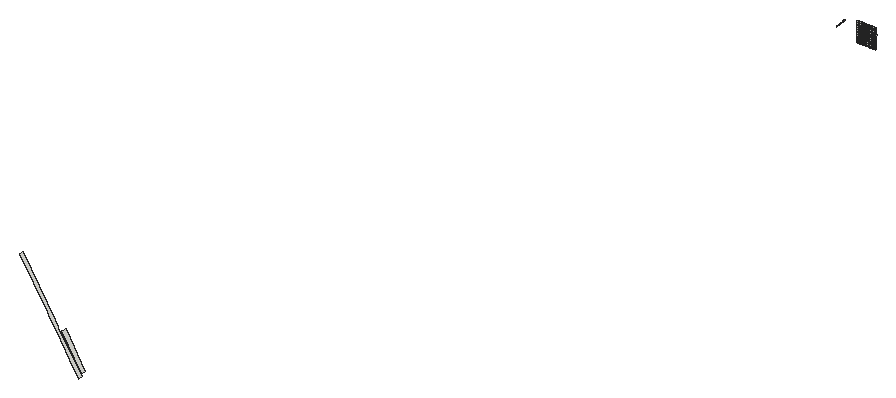
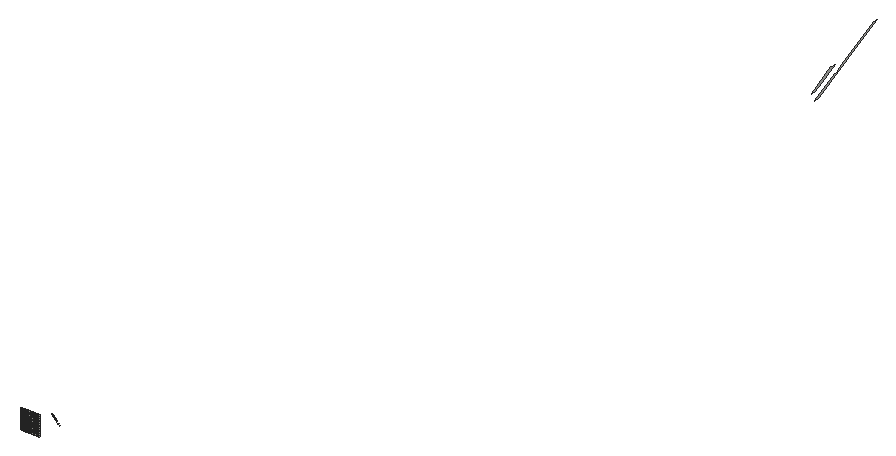
# SketchUp Ruby script. Lengths in inches.
U = 1.inch
M = Sketchup.active_model
def pt(a) = Geom::Point3d.new(a.map { |v| v * U })
def face(e, loops, mat)
  f = e.add_face(loops[0].map { |a| pt(a) })
  loops[1..].each { |l| e.add_face(l.map { |a| pt(a) }).erase! }
  f.material = f.back_material = mat if mat
  f
end
# faces: each face lists its corners as indices into pts; further lists are holes
def faces(e, pts, list, mat = nil) = list.each { |f| face(e, (f[0].is_a?(Array) ? f : [f]).map { |l| l.map { |i| pts[i] } }, mat) }
# xy, xz, yz: faces in a plane at the given z, y or x. An outline is a flat list of corners, or four numbers for a rectangle; further outlines are holes
def ring(l) = l.size == 4 ? [[l[0], l[1]], [l[2], l[1]], [l[2], l[3]], [l[0], l[3]]] : l.each_slice(2).to_a
def flat(e, list, mat, &to3) = list.each { |f| face(e, (f[0].is_a?(Array) ? f : [f]).map { |l| ring(l).map { |u, v| to3.(u, v) } }, mat) }
def xy(e, z, list, mat = nil) = flat(e, list, mat) { |x, y| [x, y, z] }
def xz(e, y, list, mat = nil) = flat(e, list, mat) { |x, z| [x, y, z] }
def yz(e, x, list, mat = nil) = flat(e, list, mat) { |y, z| [x, y, z] }
def lines(e, pts, list) = list.each { |a, b| e.add_line(pt(pts[a]), pt(pts[b])) }
# prism: a flat outline (further loops are holes) pulled along v
def prism(e, loops, v, mat = nil)
  f = face(e, loops, mat); d = Geom::Vector3d.new(v.map { |x| x * U })
  f.pushpull(f.normal.samedirection?(d) ? d.length : -d.length)
end
def box(e, o, s, mat = nil) = prism(e, [[o, [o[0] + s[0], o[1], o[2]], [o[0] + s[0], o[1] + s[1], o[2]], [o[0], o[1] + s[1], o[2]]]], [0, 0, s[2]], mat)
def at(x, y, z, deg = 0) = Geom::Transformation.translation(pt([x, y, z])) * Geom::Transformation.rotation(ORIGIN, Z_AXIS, deg.degrees)
def axes(o, x, y, z) = Geom::Transformation.new([*x, 0, *y, 0, *z, 0, *pt(o).to_a, 1])
def part(name) = M.definitions.add(name)
# library, detail: a bought-in or finely detailed component or shape, given as its bounding box
def library(name, o, s) = part(name).tap { |d| box(d.entities, o, s) }
def detail(e, o, s) = box(e.add_group.entities, o, s)
def put(e, d, t, mat = nil) = e.add_instance(d, t).tap { |i| i.material = mat if mat }
def group(e, t, mat = nil) = e.add_group.tap { |g| g.transformation = t; g.material = mat if mat }.entities
root = M.entities
M.materials.add("[Color M06]").color = [79, 71, 84]
xy(root,265.77,[[951.52,2332.13,953.84,2332.76],[954.4375,2332.13,956.75,2332.76],[957.35,2332.13,959.66,2332.76],[960.26,2332.13,962.57,2332.76],[963.17,2332.13,965.48,2332.76],
  [966.08,2332.13,968.4,2332.76],[969,2332.13,971.31,2332.76],[971.91,2332.13,974.22,2332.76],[974.82,2332.13,977.13,2332.76],[977.73,2332.13,980.04,2332.76],
  [980.64,2332.13,982.96,2332.76],[983.56,2332.13,985.87,2332.76],[986.47,2332.13,988.78,2332.76]])
xy(root,268.09,[[951.52,2332.13,953.84,2332.76],[954.4375,2332.13,956.75,2332.76],[957.35,2332.13,959.66,2332.76],[960.26,2332.13,962.57,2332.76],[963.17,2332.13,965.48,2332.76],
  [966.08,2332.13,968.4,2332.76],[969,2332.13,971.31,2332.76],[971.91,2332.13,974.22,2332.76],[974.82,2332.13,977.13,2332.76],[977.73,2332.13,980.04,2332.76],
  [980.64,2332.13,982.96,2332.76],[983.56,2332.13,985.87,2332.76],[986.47,2332.13,988.78,2332.76]])
xy(root,268.82,[[951.55,2332.13,953.87,2332.76],[954.46,2332.13,956.78,2332.76],[957.38,2332.13,959.69,2332.76],[960.29,2332.13,962.6,2332.76],[963.2,2332.13,965.51,2332.76],
  [966.11,2332.13,968.43,2332.76],[969.03,2332.13,971.34,2332.76],[971.9375,2332.13,974.25,2332.76],[974.85,2332.13,977.16,2332.76],[977.76,2332.13,980.07,2332.76],
  [980.67,2332.13,982.99,2332.76],[983.59,2332.13,985.9,2332.76],[986.5,2332.13,988.81,2332.76]])
xy(root,271.13,[[951.55,2332.13,953.87,2332.76],[954.46,2332.13,956.78,2332.76],[957.38,2332.13,959.69,2332.76],[960.29,2332.13,962.6,2332.76],[963.2,2332.13,965.51,2332.76],
  [966.11,2332.13,968.43,2332.76],[969.03,2332.13,971.34,2332.76],[971.9375,2332.13,974.25,2332.76],[974.85,2332.13,977.16,2332.76],[977.76,2332.13,980.07,2332.76],
  [980.67,2332.13,982.99,2332.76],[983.59,2332.13,985.9,2332.76],[986.5,2332.13,988.81,2332.76]])
xy(root,271.86,[[951.58,2332.13,953.89,2332.76],[954.49,2332.13,956.81,2332.76],[957.41,2332.13,959.72,2332.76],[960.32,2332.13,962.63,2332.76],[963.23,2332.13,965.54,2332.76],
  [966.14,2332.13,968.45,2332.76],[969.05,2332.13,971.37,2332.76],[971.97,2332.13,974.28,2332.76],[974.88,2332.13,977.19,2332.76],[977.79,2332.13,980.1,2332.76],
  [980.7,2332.13,983.01,2332.76],[983.61,2332.13,985.93,2332.76],[986.53,2332.13,988.84,2332.76]])
xy(root,274.17,[[951.58,2332.13,953.89,2332.76],[954.49,2332.13,956.81,2332.76],[957.41,2332.13,959.72,2332.76],[960.32,2332.13,962.63,2332.76],[963.23,2332.13,965.54,2332.76],
  [966.14,2332.13,968.45,2332.76],[969.05,2332.13,971.37,2332.76],[971.97,2332.13,974.28,2332.76],[974.88,2332.13,977.19,2332.76],[977.79,2332.13,980.1,2332.76],
  [980.7,2332.13,983.01,2332.76],[983.61,2332.13,985.93,2332.76],[986.53,2332.13,988.84,2332.76]])
xy(root,274.91,[[951.61,2332.13,953.92,2332.76],[954.52,2332.13,956.84,2332.76],[957.44,2332.13,959.75,2332.76],[960.35,2332.13,962.66,2332.76],[963.26,2332.13,965.57,2332.76],
  [966.17,2332.13,968.48,2332.76],[969.08,2332.13,971.4,2332.76],[972,2332.13,974.31,2332.76],[974.91,2332.13,977.22,2332.76],[977.82,2332.13,980.13,2332.76],
  [980.73,2332.13,983.04,2332.76],[983.64,2332.13,985.96,2332.76],[986.56,2332.13,988.87,2332.76]])
xy(root,277.22,[[951.61,2332.13,953.92,2332.76],[954.52,2332.13,956.84,2332.76],[957.44,2332.13,959.75,2332.76],[960.35,2332.13,962.66,2332.76],[963.26,2332.13,965.57,2332.76],
  [966.17,2332.13,968.48,2332.76],[969.08,2332.13,971.4,2332.76],[972,2332.13,974.31,2332.76],[974.91,2332.13,977.22,2332.76],[977.82,2332.13,980.13,2332.76],
  [980.73,2332.13,983.04,2332.76],[983.64,2332.13,985.96,2332.76],[986.56,2332.13,988.87,2332.76]])
xy(root,277.95,[[951.64,2332.13,953.95,2332.76],[954.55,2332.13,956.86,2332.76],[957.46,2332.13,959.78,2332.76],[960.375,2332.13,962.6875,2332.76],[963.29,2332.13,965.6,2332.76],
  [966.2,2332.13,968.51,2332.76],[969.11,2332.13,971.42,2332.76],[972.02,2332.13,974.34,2332.76],[974.9375,2332.13,977.25,2332.76],[977.85,2332.13,980.16,2332.76],
  [980.76,2332.13,983.07,2332.76],[983.67,2332.13,985.98,2332.76],[986.58,2332.13,988.9,2332.76]])
xy(root,280.26,[[951.64,2332.13,953.95,2332.76],[954.55,2332.13,956.86,2332.76],[957.46,2332.13,959.78,2332.76],[960.375,2332.13,962.6875,2332.76],[963.29,2332.13,965.6,2332.76],
  [966.2,2332.13,968.51,2332.76],[969.11,2332.13,971.42,2332.76],[972.02,2332.13,974.34,2332.76],[974.9375,2332.13,977.25,2332.76],[977.85,2332.13,980.16,2332.76],
  [980.76,2332.13,983.07,2332.76],[983.67,2332.13,985.98,2332.76],[986.58,2332.13,988.9,2332.76]])
xy(root,281,[[951.67,2332.13,953.98,2332.76],[954.58,2332.13,956.89,2332.76],[957.49,2332.13,959.81,2332.76],[960.41,2332.13,962.72,2332.76],[963.32,2332.13,965.63,2332.76],
  [966.23,2332.13,968.54,2332.76],[969.14,2332.13,971.45,2332.76],[972.05,2332.13,974.37,2332.76],[974.97,2332.13,977.28,2332.76],[977.88,2332.13,980.19,2332.76],
  [980.79,2332.13,983.1,2332.76],[983.7,2332.13,986.01,2332.76],[986.61,2332.13,988.93,2332.76]])
xy(root,283.31,[[951.67,2332.13,953.98,2332.76],[954.58,2332.13,956.89,2332.76],[957.49,2332.13,959.81,2332.76],[960.41,2332.13,962.72,2332.76],[963.32,2332.13,965.63,2332.76],
  [966.23,2332.13,968.54,2332.76],[969.14,2332.13,971.45,2332.76],[972.05,2332.13,974.37,2332.76],[974.97,2332.13,977.28,2332.76],[977.88,2332.13,980.19,2332.76],
  [980.79,2332.13,983.1,2332.76],[983.7,2332.13,986.01,2332.76],[986.61,2332.13,988.93,2332.76]])
xy(root,284.04,[[951.7,2332.13,954.01,2332.76],[954.61,2332.13,956.92,2332.76],[957.52,2332.13,959.83,2332.76],[960.43,2332.13,962.75,2332.76],[963.35,2332.13,965.66,2332.76],
  [966.26,2332.13,968.57,2332.76],[969.17,2332.13,971.48,2332.76],[972.08,2332.13,974.39,2332.76],[974.99,2332.13,977.31,2332.76],[977.91,2332.13,980.22,2332.76],
  [980.82,2332.13,983.13,2332.76],[983.73,2332.13,986.04,2332.76],[986.64,2332.13,988.95,2332.76]])
xy(root,286.35,[[951.7,2332.13,954.01,2332.76],[954.61,2332.13,956.92,2332.76],[957.52,2332.13,959.83,2332.76],[960.43,2332.13,962.75,2332.76],[963.35,2332.13,965.66,2332.76],
  [966.26,2332.13,968.57,2332.76],[969.17,2332.13,971.48,2332.76],[972.08,2332.13,974.39,2332.76],[974.99,2332.13,977.31,2332.76],[977.91,2332.13,980.22,2332.76],
  [980.82,2332.13,983.13,2332.76],[983.73,2332.13,986.04,2332.76],[986.64,2332.13,988.95,2332.76]])
xy(root,287.09,[[951.73,2332.13,954.04,2332.76],[954.64,2332.13,956.95,2332.76],[957.55,2332.13,959.86,2332.76],[960.46,2332.13,962.78,2332.76],[963.375,2332.13,965.6875,2332.76],
  [966.29,2332.13,968.6,2332.76],[969.2,2332.13,971.51,2332.76],[972.11,2332.13,974.42,2332.76],[975.02,2332.13,977.34,2332.76],[977.94,2332.13,980.25,2332.76],
  [980.85,2332.13,983.16,2332.76],[983.76,2332.13,986.07,2332.76],[986.67,2332.13,988.98,2332.76]])
xy(root,289.4,[[951.73,2332.13,954.04,2332.76],[954.64,2332.13,956.95,2332.76],[957.55,2332.13,959.86,2332.76],[960.46,2332.13,962.78,2332.76],[963.375,2332.13,965.6875,2332.76],
  [966.29,2332.13,968.6,2332.76],[969.2,2332.13,971.51,2332.76],[972.11,2332.13,974.42,2332.76],[975.02,2332.13,977.34,2332.76],[977.94,2332.13,980.25,2332.76],
  [980.85,2332.13,983.16,2332.76],[983.76,2332.13,986.07,2332.76],[986.67,2332.13,988.98,2332.76]])
xy(root,290.13,[[951.76,2332.13,954.07,2332.76],[954.67,2332.13,956.98,2332.76],[957.58,2332.13,959.89,2332.76],[960.49,2332.13,962.8,2332.76],[963.4,2332.13,965.72,2332.76],
  [966.32,2332.13,968.63,2332.76],[969.23,2332.13,971.54,2332.76],[972.14,2332.13,974.45,2332.76],[975.05,2332.13,977.36,2332.76],[977.96,2332.13,980.28,2332.76],
  [980.875,2332.13,983.1875,2332.76],[983.79,2332.13,986.1,2332.76],[986.7,2332.13,989.01,2332.76]])
xy(root,292.44,[[951.76,2332.13,954.07,2332.76],[954.67,2332.13,956.98,2332.76],[957.58,2332.13,959.89,2332.76],[960.49,2332.13,962.8,2332.76],[963.4,2332.13,965.72,2332.76],
  [966.32,2332.13,968.63,2332.76],[969.23,2332.13,971.54,2332.76],[972.14,2332.13,974.45,2332.76],[975.05,2332.13,977.36,2332.76],[977.96,2332.13,980.28,2332.76],
  [980.875,2332.13,983.1875,2332.76],[983.79,2332.13,986.1,2332.76],[986.7,2332.13,989.01,2332.76]])
xy(root,293.18,[[951.78,2332.13,954.1,2332.76],[954.7,2332.13,957.01,2332.76],[957.61,2332.13,959.92,2332.76],[960.52,2332.13,962.83,2332.76],[963.43,2332.13,965.75,2332.76],
  [966.35,2332.13,968.66,2332.76],[969.26,2332.13,971.57,2332.76],[972.17,2332.13,974.48,2332.76],[975.08,2332.13,977.39,2332.76],[977.99,2332.13,980.31,2332.76],
  [980.91,2332.13,983.22,2332.76],[983.82,2332.13,986.13,2332.76],[986.73,2332.13,989.04,2332.76]])
xy(root,295.49,[[951.78,2332.13,954.1,2332.76],[954.7,2332.13,957.01,2332.76],[957.61,2332.13,959.92,2332.76],[960.52,2332.13,962.83,2332.76],[963.43,2332.13,965.75,2332.76],
  [966.35,2332.13,968.66,2332.76],[969.26,2332.13,971.57,2332.76],[972.17,2332.13,974.48,2332.76],[975.08,2332.13,977.39,2332.76],[977.99,2332.13,980.31,2332.76],
  [980.91,2332.13,983.22,2332.76],[983.82,2332.13,986.13,2332.76],[986.73,2332.13,989.04,2332.76]])
xy(root,296.22,[[951.8125,2332.13,954.125,2332.76],[954.73,2332.13,957.04,2332.76],[957.64,2332.13,959.95,2332.76],[960.55,2332.13,962.86,2332.76],[963.46,2332.13,965.77,2332.76],
  [966.375,2332.13,968.6875,2332.76],[969.29,2332.13,971.6,2332.76],[972.2,2332.13,974.51,2332.76],[975.11,2332.13,977.42,2332.76],[978.02,2332.13,980.33,2332.76],
  [980.93,2332.13,983.25,2332.76],[983.85,2332.13,986.16,2332.76],[986.76,2332.13,989.07,2332.76]])
xy(root,298.53,[[951.8125,2332.13,954.125,2332.76],[954.73,2332.13,957.04,2332.76],[957.64,2332.13,959.95,2332.76],[960.55,2332.13,962.86,2332.76],[963.46,2332.13,965.77,2332.76],
  [966.375,2332.13,968.6875,2332.76],[969.29,2332.13,971.6,2332.76],[972.2,2332.13,974.51,2332.76],[975.11,2332.13,977.42,2332.76],[978.02,2332.13,980.33,2332.76],
  [980.93,2332.13,983.25,2332.76],[983.85,2332.13,986.16,2332.76],[986.76,2332.13,989.07,2332.76]])
xy(root,299.27,[[951.84,2332.13,954.16,2332.76],[954.75,2332.13,957.07,2332.76],[957.67,2332.13,959.98,2332.76],[960.58,2332.13,962.89,2332.76],[963.49,2332.13,965.8,2332.76],
  [966.4,2332.13,968.72,2332.76],[969.32,2332.13,971.63,2332.76],[972.23,2332.13,974.54,2332.76],[975.14,2332.13,977.45,2332.76],[978.05,2332.13,980.36,2332.76],
  [980.96,2332.13,983.28,2332.76],[983.875,2332.13,986.1875,2332.76],[986.79,2332.13,989.1,2332.76]])
xy(root,301.58,[[951.84,2332.13,954.16,2332.76],[954.75,2332.13,957.07,2332.76],[957.67,2332.13,959.98,2332.76],[960.58,2332.13,962.89,2332.76],[963.49,2332.13,965.8,2332.76],
  [966.4,2332.13,968.72,2332.76],[969.32,2332.13,971.63,2332.76],[972.23,2332.13,974.54,2332.76],[975.14,2332.13,977.45,2332.76],[978.05,2332.13,980.36,2332.76],
  [980.96,2332.13,983.28,2332.76],[983.875,2332.13,986.1875,2332.76],[986.79,2332.13,989.1,2332.76]])
xy(root,302.31,[[951.87,2332.13,954.18,2332.76],[954.78,2332.13,957.1,2332.76],[957.7,2332.13,960.01,2332.76],[960.61,2332.13,962.92,2332.76],[963.52,2332.13,965.83,2332.76],
  [966.43,2332.13,968.74,2332.76],[969.34,2332.13,971.66,2332.76],[972.26,2332.13,974.57,2332.76],[975.17,2332.13,977.48,2332.76],[978.08,2332.13,980.39,2332.76],
  [980.99,2332.13,983.3,2332.76],[983.9,2332.13,986.22,2332.76],[986.82,2332.13,989.13,2332.76]])
xy(root,304.62,[[951.87,2332.13,954.18,2332.76],[954.78,2332.13,957.1,2332.76],[957.7,2332.13,960.01,2332.76],[960.61,2332.13,962.92,2332.76],[963.52,2332.13,965.83,2332.76],
  [966.43,2332.13,968.74,2332.76],[969.34,2332.13,971.66,2332.76],[972.26,2332.13,974.57,2332.76],[975.17,2332.13,977.48,2332.76],[978.08,2332.13,980.39,2332.76],
  [980.99,2332.13,983.3,2332.76],[983.9,2332.13,986.22,2332.76],[986.82,2332.13,989.13,2332.76]])
xz(root,2319.18,[[921.31,289.13,923.73,291.7,923.27,292.13,920.85,289.56],[924.61,292.64,927.03,295.21,926.57,295.64,924.15,293.0625],[927.91,296.14,930.33,298.71,929.87,299.14,927.45,296.57],[931.2,299.64,933.625,302.22,933.17,302.64,930.75,300.07],[934.5,303.15,936.92,305.72,936.47,306.15,934.05,303.58],
  [934.05,303.58,936.47,306.15,936.24,306.36,933.82,303.79]],"[Color M06]")
yz(root,951.52,[[2332.13,265.77,2332.76,268.09]])
yz(root,951.55,[[2332.13,268.82,2332.76,271.13]])
yz(root,951.58,[[2332.13,271.86,2332.76,274.17]])
yz(root,951.61,[[2332.13,274.91,2332.76,277.22]])
yz(root,951.64,[[2332.13,277.95,2332.76,280.26]])
yz(root,951.67,[[2332.13,281,2332.76,283.31]])
yz(root,951.7,[[2332.13,284.04,2332.76,286.35]])
yz(root,951.73,[[2332.13,287.09,2332.76,289.4]])
yz(root,951.76,[[2332.13,290.13,2332.76,292.44]])
yz(root,951.78,[[2332.13,293.18,2332.76,295.49]])
yz(root,951.8125,[[2332.13,296.22,2332.76,298.53]])
yz(root,951.84,[[2332.13,299.27,2332.76,301.58]])
yz(root,951.87,[[2332.13,302.31,2332.76,304.62]])
yz(root,953.84,[[2332.13,265.77,2332.76,268.09]])
yz(root,953.87,[[2332.13,268.82,2332.76,271.13]])
yz(root,953.89,[[2332.13,271.86,2332.76,274.17]])
yz(root,953.92,[[2332.13,274.91,2332.76,277.22]])
yz(root,953.95,[[2332.13,277.95,2332.76,280.26]])
yz(root,953.98,[[2332.13,281,2332.76,283.31]])
yz(root,954.01,[[2332.13,284.04,2332.76,286.35]])
yz(root,954.04,[[2332.13,287.09,2332.76,289.4]])
yz(root,954.07,[[2332.13,290.13,2332.76,292.44]])
yz(root,954.1,[[2332.13,293.18,2332.76,295.49]])
yz(root,954.125,[[2332.13,296.22,2332.76,298.53]])
yz(root,954.16,[[2332.13,299.27,2332.76,301.58]])
yz(root,954.18,[[2332.13,302.31,2332.76,304.62]])
yz(root,954.4375,[[2332.13,265.77,2332.76,268.09]])
yz(root,954.46,[[2332.13,268.82,2332.76,271.13]])
yz(root,954.49,[[2332.13,271.86,2332.76,274.17]])
yz(root,954.52,[[2332.13,274.91,2332.76,277.22]])
yz(root,954.55,[[2332.13,277.95,2332.76,280.26]])
yz(root,954.58,[[2332.13,281,2332.76,283.31]])
yz(root,954.61,[[2332.13,284.04,2332.76,286.35]])
yz(root,954.64,[[2332.13,287.09,2332.76,289.4]])
yz(root,954.67,[[2332.13,290.13,2332.76,292.44]])
yz(root,954.7,[[2332.13,293.18,2332.76,295.49]])
yz(root,954.73,[[2332.13,296.22,2332.76,298.53]])
yz(root,954.75,[[2332.13,299.27,2332.76,301.58]])
yz(root,954.78,[[2332.13,302.31,2332.76,304.62]])
yz(root,956.75,[[2332.13,265.77,2332.76,268.09]])
yz(root,956.78,[[2332.13,268.82,2332.76,271.13]])
yz(root,956.81,[[2332.13,271.86,2332.76,274.17]])
yz(root,956.84,[[2332.13,274.91,2332.76,277.22]])
yz(root,956.86,[[2332.13,277.95,2332.76,280.26]])
yz(root,956.89,[[2332.13,281,2332.76,283.31]])
yz(root,956.92,[[2332.13,284.04,2332.76,286.35]])
yz(root,956.95,[[2332.13,287.09,2332.76,289.4]])
yz(root,956.98,[[2332.13,290.13,2332.76,292.44]])
yz(root,957.01,[[2332.13,293.18,2332.76,295.49]])
yz(root,957.04,[[2332.13,296.22,2332.76,298.53]])
yz(root,957.07,[[2332.13,299.27,2332.76,301.58]])
yz(root,957.1,[[2332.13,302.31,2332.76,304.62]])
yz(root,957.35,[[2332.13,265.77,2332.76,268.09]])
yz(root,957.38,[[2332.13,268.82,2332.76,271.13]])
yz(root,957.41,[[2332.13,271.86,2332.76,274.17]])
yz(root,957.44,[[2332.13,274.91,2332.76,277.22]])
yz(root,957.46,[[2332.13,277.95,2332.76,280.26]])
yz(root,957.49,[[2332.13,281,2332.76,283.31]])
yz(root,957.52,[[2332.13,284.04,2332.76,286.35]])
yz(root,957.55,[[2332.13,287.09,2332.76,289.4]])
yz(root,957.58,[[2332.13,290.13,2332.76,292.44]])
yz(root,957.61,[[2332.13,293.18,2332.76,295.49]])
yz(root,957.64,[[2332.13,296.22,2332.76,298.53]])
yz(root,957.67,[[2332.13,299.27,2332.76,301.58]])
yz(root,957.7,[[2332.13,302.31,2332.76,304.62]])
yz(root,959.66,[[2332.13,265.77,2332.76,268.09]])
yz(root,959.69,[[2332.13,268.82,2332.76,271.13]])
yz(root,959.72,[[2332.13,271.86,2332.76,274.17]])
yz(root,959.75,[[2332.13,274.91,2332.76,277.22]])
yz(root,959.78,[[2332.13,277.95,2332.76,280.26]])
yz(root,959.81,[[2332.13,281,2332.76,283.31]])
yz(root,959.83,[[2332.13,284.04,2332.76,286.35]])
yz(root,959.86,[[2332.13,287.09,2332.76,289.4]])
yz(root,959.89,[[2332.13,290.13,2332.76,292.44]])
yz(root,959.92,[[2332.13,293.18,2332.76,295.49]])
yz(root,959.95,[[2332.13,296.22,2332.76,298.53]])
yz(root,959.98,[[2332.13,299.27,2332.76,301.58]])
yz(root,960.01,[[2332.13,302.31,2332.76,304.62]])
yz(root,960.26,[[2332.13,265.77,2332.76,268.09]])
yz(root,960.29,[[2332.13,268.82,2332.76,271.13]])
yz(root,960.32,[[2332.13,271.86,2332.76,274.17]])
yz(root,960.35,[[2332.13,274.91,2332.76,277.22]])
yz(root,960.375,[[2332.13,277.95,2332.76,280.26]])
yz(root,960.41,[[2332.13,281,2332.76,283.31]])
yz(root,960.43,[[2332.13,284.04,2332.76,286.35]])
yz(root,960.46,[[2332.13,287.09,2332.76,289.4]])
yz(root,960.49,[[2332.13,290.13,2332.76,292.44]])
yz(root,960.52,[[2332.13,293.18,2332.76,295.49]])
yz(root,960.55,[[2332.13,296.22,2332.76,298.53]])
yz(root,960.58,[[2332.13,299.27,2332.76,301.58]])
yz(root,960.61,[[2332.13,302.31,2332.76,304.62]])
yz(root,962.57,[[2332.13,265.77,2332.76,268.09]])
yz(root,962.6,[[2332.13,268.82,2332.76,271.13]])
yz(root,962.63,[[2332.13,271.86,2332.76,274.17]])
yz(root,962.66,[[2332.13,274.91,2332.76,277.22]])
yz(root,962.6875,[[2332.13,277.95,2332.76,280.26]])
yz(root,962.72,[[2332.13,281,2332.76,283.31]])
yz(root,962.75,[[2332.13,284.04,2332.76,286.35]])
yz(root,962.78,[[2332.13,287.09,2332.76,289.4]])
yz(root,962.8,[[2332.13,290.13,2332.76,292.44]])
yz(root,962.83,[[2332.13,293.18,2332.76,295.49]])
yz(root,962.86,[[2332.13,296.22,2332.76,298.53]])
yz(root,962.89,[[2332.13,299.27,2332.76,301.58]])
yz(root,962.92,[[2332.13,302.31,2332.76,304.62]])
yz(root,963.17,[[2332.13,265.77,2332.76,268.09]])
yz(root,963.2,[[2332.13,268.82,2332.76,271.13]])
yz(root,963.23,[[2332.13,271.86,2332.76,274.17]])
yz(root,963.26,[[2332.13,274.91,2332.76,277.22]])
yz(root,963.29,[[2332.13,277.95,2332.76,280.26]])
yz(root,963.32,[[2332.13,281,2332.76,283.31]])
yz(root,963.35,[[2332.13,284.04,2332.76,286.35]])
yz(root,963.375,[[2332.13,287.09,2332.76,289.4]])
yz(root,963.4,[[2332.13,290.13,2332.76,292.44]])
yz(root,963.43,[[2332.13,293.18,2332.76,295.49]])
yz(root,963.46,[[2332.13,296.22,2332.76,298.53]])
yz(root,963.49,[[2332.13,299.27,2332.76,301.58]])
yz(root,963.52,[[2332.13,302.31,2332.76,304.62]])
yz(root,965.48,[[2332.13,265.77,2332.76,268.09]])
yz(root,965.51,[[2332.13,268.82,2332.76,271.13]])
yz(root,965.54,[[2332.13,271.86,2332.76,274.17]])
yz(root,965.57,[[2332.13,274.91,2332.76,277.22]])
yz(root,965.6,[[2332.13,277.95,2332.76,280.26]])
yz(root,965.63,[[2332.13,281,2332.76,283.31]])
yz(root,965.66,[[2332.13,284.04,2332.76,286.35]])
yz(root,965.6875,[[2332.13,287.09,2332.76,289.4]])
yz(root,965.72,[[2332.13,290.13,2332.76,292.44]])
yz(root,965.75,[[2332.13,293.18,2332.76,295.49]])
yz(root,965.77,[[2332.13,296.22,2332.76,298.53]])
yz(root,965.8,[[2332.13,299.27,2332.76,301.58]])
yz(root,965.83,[[2332.13,302.31,2332.76,304.62]])
yz(root,966.08,[[2332.13,265.77,2332.76,268.09]])
yz(root,966.11,[[2332.13,268.82,2332.76,271.13]])
yz(root,966.14,[[2332.13,271.86,2332.76,274.17]])
yz(root,966.17,[[2332.13,274.91,2332.76,277.22]])
yz(root,966.2,[[2332.13,277.95,2332.76,280.26]])
yz(root,966.23,[[2332.13,281,2332.76,283.31]])
yz(root,966.26,[[2332.13,284.04,2332.76,286.35]])
yz(root,966.29,[[2332.13,287.09,2332.76,289.4]])
yz(root,966.32,[[2332.13,290.13,2332.76,292.44]])
yz(root,966.35,[[2332.13,293.18,2332.76,295.49]])
yz(root,966.375,[[2332.13,296.22,2332.76,298.53]])
yz(root,966.4,[[2332.13,299.27,2332.76,301.58]])
yz(root,966.43,[[2332.13,302.31,2332.76,304.62]])
yz(root,968.4,[[2332.13,265.77,2332.76,268.09]])
yz(root,968.43,[[2332.13,268.82,2332.76,271.13]])
yz(root,968.45,[[2332.13,271.86,2332.76,274.17]])
yz(root,968.48,[[2332.13,274.91,2332.76,277.22]])
yz(root,968.51,[[2332.13,277.95,2332.76,280.26]])
yz(root,968.54,[[2332.13,281,2332.76,283.31]])
yz(root,968.57,[[2332.13,284.04,2332.76,286.35]])
yz(root,968.6,[[2332.13,287.09,2332.76,289.4]])
yz(root,968.63,[[2332.13,290.13,2332.76,292.44]])
yz(root,968.66,[[2332.13,293.18,2332.76,295.49]])
yz(root,968.6875,[[2332.13,296.22,2332.76,298.53]])
yz(root,968.72,[[2332.13,299.27,2332.76,301.58]])
yz(root,968.74,[[2332.13,302.31,2332.76,304.62]])
yz(root,969,[[2332.13,265.77,2332.76,268.09]])
yz(root,969.03,[[2332.13,268.82,2332.76,271.13]])
yz(root,969.05,[[2332.13,271.86,2332.76,274.17]])
yz(root,969.08,[[2332.13,274.91,2332.76,277.22]])
yz(root,969.11,[[2332.13,277.95,2332.76,280.26]])
yz(root,969.14,[[2332.13,281,2332.76,283.31]])
yz(root,969.17,[[2332.13,284.04,2332.76,286.35]])
yz(root,969.2,[[2332.13,287.09,2332.76,289.4]])
yz(root,969.23,[[2332.13,290.13,2332.76,292.44]])
yz(root,969.26,[[2332.13,293.18,2332.76,295.49]])
yz(root,969.29,[[2332.13,296.22,2332.76,298.53]])
yz(root,969.32,[[2332.13,299.27,2332.76,301.58]])
yz(root,969.34,[[2332.13,302.31,2332.76,304.62]])
yz(root,971.31,[[2332.13,265.77,2332.76,268.09]])
yz(root,971.34,[[2332.13,268.82,2332.76,271.13]])
yz(root,971.37,[[2332.13,271.86,2332.76,274.17]])
yz(root,971.4,[[2332.13,274.91,2332.76,277.22]])
yz(root,971.42,[[2332.13,277.95,2332.76,280.26]])
yz(root,971.45,[[2332.13,281,2332.76,283.31]])
yz(root,971.48,[[2332.13,284.04,2332.76,286.35]])
yz(root,971.51,[[2332.13,287.09,2332.76,289.4]])
yz(root,971.54,[[2332.13,290.13,2332.76,292.44]])
yz(root,971.57,[[2332.13,293.18,2332.76,295.49]])
yz(root,971.6,[[2332.13,296.22,2332.76,298.53]])
yz(root,971.63,[[2332.13,299.27,2332.76,301.58]])
yz(root,971.66,[[2332.13,302.31,2332.76,304.62]])
yz(root,971.91,[[2332.13,265.77,2332.76,268.09]])
yz(root,971.9375,[[2332.13,268.82,2332.76,271.13]])
yz(root,971.97,[[2332.13,271.86,2332.76,274.17]])
yz(root,972,[[2332.13,274.91,2332.76,277.22]])
yz(root,972.02,[[2332.13,277.95,2332.76,280.26]])
yz(root,972.05,[[2332.13,281,2332.76,283.31]])
yz(root,972.08,[[2332.13,284.04,2332.76,286.35]])
yz(root,972.11,[[2332.13,287.09,2332.76,289.4]])
yz(root,972.14,[[2332.13,290.13,2332.76,292.44]])
yz(root,972.17,[[2332.13,293.18,2332.76,295.49]])
yz(root,972.2,[[2332.13,296.22,2332.76,298.53]])
yz(root,972.23,[[2332.13,299.27,2332.76,301.58]])
yz(root,972.26,[[2332.13,302.31,2332.76,304.62]])
yz(root,974.22,[[2332.13,265.77,2332.76,268.09]])
yz(root,974.25,[[2332.13,268.82,2332.76,271.13]])
yz(root,974.28,[[2332.13,271.86,2332.76,274.17]])
yz(root,974.31,[[2332.13,274.91,2332.76,277.22]])
yz(root,974.34,[[2332.13,277.95,2332.76,280.26]])
yz(root,974.37,[[2332.13,281,2332.76,283.31]])
yz(root,974.39,[[2332.13,284.04,2332.76,286.35]])
yz(root,974.42,[[2332.13,287.09,2332.76,289.4]])
yz(root,974.45,[[2332.13,290.13,2332.76,292.44]])
yz(root,974.48,[[2332.13,293.18,2332.76,295.49]])
yz(root,974.51,[[2332.13,296.22,2332.76,298.53]])
yz(root,974.54,[[2332.13,299.27,2332.76,301.58]])
yz(root,974.57,[[2332.13,302.31,2332.76,304.62]])
yz(root,974.82,[[2332.13,265.77,2332.76,268.09]])
yz(root,974.85,[[2332.13,268.82,2332.76,271.13]])
yz(root,974.88,[[2332.13,271.86,2332.76,274.17]])
yz(root,974.91,[[2332.13,274.91,2332.76,277.22]])
yz(root,974.9375,[[2332.13,277.95,2332.76,280.26]])
yz(root,974.97,[[2332.13,281,2332.76,283.31]])
yz(root,974.99,[[2332.13,284.04,2332.76,286.35]])
yz(root,975.02,[[2332.13,287.09,2332.76,289.4]])
yz(root,975.05,[[2332.13,290.13,2332.76,292.44]])
yz(root,975.08,[[2332.13,293.18,2332.76,295.49]])
yz(root,975.11,[[2332.13,296.22,2332.76,298.53]])
yz(root,975.14,[[2332.13,299.27,2332.76,301.58]])
yz(root,975.17,[[2332.13,302.31,2332.76,304.62]])
yz(root,977.13,[[2332.13,265.77,2332.76,268.09]])
yz(root,977.16,[[2332.13,268.82,2332.76,271.13]])
yz(root,977.19,[[2332.13,271.86,2332.76,274.17]])
yz(root,977.22,[[2332.13,274.91,2332.76,277.22]])
yz(root,977.25,[[2332.13,277.95,2332.76,280.26]])
yz(root,977.28,[[2332.13,281,2332.76,283.31]])
yz(root,977.31,[[2332.13,284.04,2332.76,286.35]])
yz(root,977.34,[[2332.13,287.09,2332.76,289.4]])
yz(root,977.36,[[2332.13,290.13,2332.76,292.44]])
yz(root,977.39,[[2332.13,293.18,2332.76,295.49]])
yz(root,977.42,[[2332.13,296.22,2332.76,298.53]])
yz(root,977.45,[[2332.13,299.27,2332.76,301.58]])
yz(root,977.48,[[2332.13,302.31,2332.76,304.62]])
yz(root,977.73,[[2332.13,265.77,2332.76,268.09]])
yz(root,977.76,[[2332.13,268.82,2332.76,271.13]])
yz(root,977.79,[[2332.13,271.86,2332.76,274.17]])
yz(root,977.82,[[2332.13,274.91,2332.76,277.22]])
yz(root,977.85,[[2332.13,277.95,2332.76,280.26]])
yz(root,977.88,[[2332.13,281,2332.76,283.31]])
yz(root,977.91,[[2332.13,284.04,2332.76,286.35]])
yz(root,977.94,[[2332.13,287.09,2332.76,289.4]])
yz(root,977.96,[[2332.13,290.13,2332.76,292.44]])
yz(root,977.99,[[2332.13,293.18,2332.76,295.49]])
yz(root,978.02,[[2332.13,296.22,2332.76,298.53]])
yz(root,978.05,[[2332.13,299.27,2332.76,301.58]])
yz(root,978.08,[[2332.13,302.31,2332.76,304.62]])
yz(root,980.04,[[2332.13,265.77,2332.76,268.09]])
yz(root,980.07,[[2332.13,268.82,2332.76,271.13]])
yz(root,980.1,[[2332.13,271.86,2332.76,274.17]])
yz(root,980.13,[[2332.13,274.91,2332.76,277.22]])
yz(root,980.16,[[2332.13,277.95,2332.76,280.26]])
yz(root,980.19,[[2332.13,281,2332.76,283.31]])
yz(root,980.22,[[2332.13,284.04,2332.76,286.35]])
yz(root,980.25,[[2332.13,287.09,2332.76,289.4]])
yz(root,980.28,[[2332.13,290.13,2332.76,292.44]])
yz(root,980.31,[[2332.13,293.18,2332.76,295.49]])
yz(root,980.33,[[2332.13,296.22,2332.76,298.53]])
yz(root,980.36,[[2332.13,299.27,2332.76,301.58]])
yz(root,980.39,[[2332.13,302.31,2332.76,304.62]])
yz(root,980.64,[[2332.13,265.77,2332.76,268.09]])
yz(root,980.67,[[2332.13,268.82,2332.76,271.13]])
yz(root,980.7,[[2332.13,271.86,2332.76,274.17]])
yz(root,980.73,[[2332.13,274.91,2332.76,277.22]])
yz(root,980.76,[[2332.13,277.95,2332.76,280.26]])
yz(root,980.79,[[2332.13,281,2332.76,283.31]])
yz(root,980.82,[[2332.13,284.04,2332.76,286.35]])
yz(root,980.85,[[2332.13,287.09,2332.76,289.4]])
yz(root,980.875,[[2332.13,290.13,2332.76,292.44]])
yz(root,980.91,[[2332.13,293.18,2332.76,295.49]])
yz(root,980.93,[[2332.13,296.22,2332.76,298.53]])
yz(root,980.96,[[2332.13,299.27,2332.76,301.58]])
yz(root,980.99,[[2332.13,302.31,2332.76,304.62]])
yz(root,982.96,[[2332.13,265.77,2332.76,268.09]])
yz(root,982.99,[[2332.13,268.82,2332.76,271.13]])
yz(root,983.01,[[2332.13,271.86,2332.76,274.17]])
yz(root,983.04,[[2332.13,274.91,2332.76,277.22]])
yz(root,983.07,[[2332.13,277.95,2332.76,280.26]])
yz(root,983.1,[[2332.13,281,2332.76,283.31]])
yz(root,983.13,[[2332.13,284.04,2332.76,286.35]])
yz(root,983.16,[[2332.13,287.09,2332.76,289.4]])
yz(root,983.1875,[[2332.13,290.13,2332.76,292.44]])
yz(root,983.22,[[2332.13,293.18,2332.76,295.49]])
yz(root,983.25,[[2332.13,296.22,2332.76,298.53]])
yz(root,983.28,[[2332.13,299.27,2332.76,301.58]])
yz(root,983.3,[[2332.13,302.31,2332.76,304.62]])
yz(root,983.56,[[2332.13,265.77,2332.76,268.09]])
yz(root,983.59,[[2332.13,268.82,2332.76,271.13]])
yz(root,983.61,[[2332.13,271.86,2332.76,274.17]])
yz(root,983.64,[[2332.13,274.91,2332.76,277.22]])
yz(root,983.67,[[2332.13,277.95,2332.76,280.26]])
yz(root,983.7,[[2332.13,281,2332.76,283.31]])
yz(root,983.73,[[2332.13,284.04,2332.76,286.35]])
yz(root,983.76,[[2332.13,287.09,2332.76,289.4]])
yz(root,983.79,[[2332.13,290.13,2332.76,292.44]])
yz(root,983.82,[[2332.13,293.18,2332.76,295.49]])
yz(root,983.85,[[2332.13,296.22,2332.76,298.53]])
yz(root,983.875,[[2332.13,299.27,2332.76,301.58]])
yz(root,983.9,[[2332.13,302.31,2332.76,304.62]])
yz(root,985.87,[[2332.13,265.77,2332.76,268.09]])
yz(root,985.9,[[2332.13,268.82,2332.76,271.13]])
yz(root,985.93,[[2332.13,271.86,2332.76,274.17]])
yz(root,985.96,[[2332.13,274.91,2332.76,277.22]])
yz(root,985.98,[[2332.13,277.95,2332.76,280.26]])
yz(root,986.01,[[2332.13,281,2332.76,283.31]])
yz(root,986.04,[[2332.13,284.04,2332.76,286.35]])
yz(root,986.07,[[2332.13,287.09,2332.76,289.4]])
yz(root,986.1,[[2332.13,290.13,2332.76,292.44]])
yz(root,986.13,[[2332.13,293.18,2332.76,295.49]])
yz(root,986.16,[[2332.13,296.22,2332.76,298.53]])
yz(root,986.1875,[[2332.13,299.27,2332.76,301.58]])
yz(root,986.22,[[2332.13,302.31,2332.76,304.62]])
yz(root,986.47,[[2332.13,265.77,2332.76,268.09]])
yz(root,986.5,[[2332.13,268.82,2332.76,271.13]])
yz(root,986.53,[[2332.13,271.86,2332.76,274.17]])
yz(root,986.56,[[2332.13,274.91,2332.76,277.22]])
yz(root,986.58,[[2332.13,277.95,2332.76,280.26]])
yz(root,986.61,[[2332.13,281,2332.76,283.31]])
yz(root,986.64,[[2332.13,284.04,2332.76,286.35]])
yz(root,986.67,[[2332.13,287.09,2332.76,289.4]])
yz(root,986.7,[[2332.13,290.13,2332.76,292.44]])
yz(root,986.73,[[2332.13,293.18,2332.76,295.49]])
yz(root,986.76,[[2332.13,296.22,2332.76,298.53]])
yz(root,986.79,[[2332.13,299.27,2332.76,301.58]])
yz(root,986.82,[[2332.13,302.31,2332.76,304.62]])
yz(root,988.78,[[2332.13,265.77,2332.76,268.09]])
yz(root,988.81,[[2332.13,268.82,2332.76,271.13]])
yz(root,988.84,[[2332.13,271.86,2332.76,274.17]])
yz(root,988.87,[[2332.13,274.91,2332.76,277.22]])
yz(root,988.9,[[2332.13,277.95,2332.76,280.26]])
yz(root,988.93,[[2332.13,281,2332.76,283.31]])
yz(root,988.95,[[2332.13,284.04,2332.76,286.35]])
yz(root,988.98,[[2332.13,287.09,2332.76,289.4]])
yz(root,989.01,[[2332.13,290.13,2332.76,292.44]])
yz(root,989.04,[[2332.13,293.18,2332.76,295.49]])
yz(root,989.07,[[2332.13,296.22,2332.76,298.53]])
yz(root,989.1,[[2332.13,299.27,2332.76,301.58]])
yz(root,989.13,[[2332.13,302.31,2332.76,304.62]])
yz(root,989.38,[[2332.13,265.77,2332.76,268.09]])
yz(root,989.41,[[2332.13,268.82,2332.76,271.13]])
yz(root,989.4375,[[2332.13,271.86,2332.76,274.17]])
yz(root,989.47,[[2332.13,274.91,2332.76,277.22]])
yz(root,989.5,[[2332.13,277.95,2332.76,280.26]])
yz(root,989.53,[[2332.13,281,2332.76,283.31]])
yz(root,989.55,[[2332.13,284.04,2332.76,286.35]])
yz(root,989.58,[[2332.13,287.09,2332.76,289.4]])
yz(root,989.61,[[2332.13,290.13,2332.76,292.44]])
p = [[553.56,731.75,450.4375],[553.56,726.125,450.4375],[608.37,726.125,364.9375],[611.36,726.125,360.28],[617.83,726.125,350.1875],[624.28,726.125,340.125],
  [663.69,726.125,278.65],[669.77,726.125,269.17],[671.46,726.125,266.53],[671.46,732.2,266.53],[632.05,732.2,328],[630.97,732.2,329.69],
  [625.08,732.2,338.875],[624.28,732.2,340.125],[623.54,732.2,341.27],[617.83,732.2,350.1875],[553.56,732.2,450.4375],[663.69,726.125,299.15],
  [637.42,726.125,340.125],[637.42,732.2,340.125],[637.42,734.4375,340.125],[677.53,734.4375,277.56],[677.53,726.125,277.56],[673.19,726.125,284.33],
  [669.77,726.125,289.67]]
faces(root,p,[[0,1,2,3,4,5,6,7,8,9,10,11,12,13,14,15,16],[17,18,19,20,21,22,23,24]])
